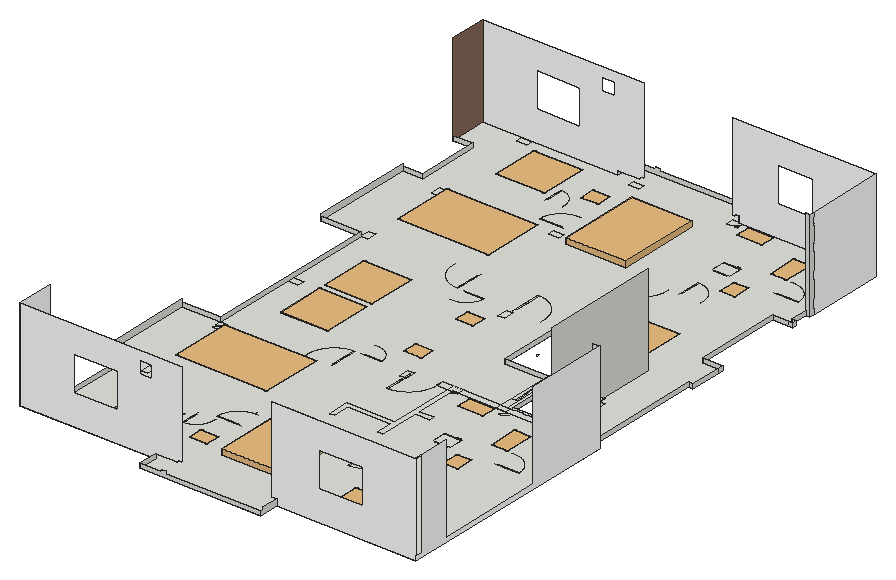
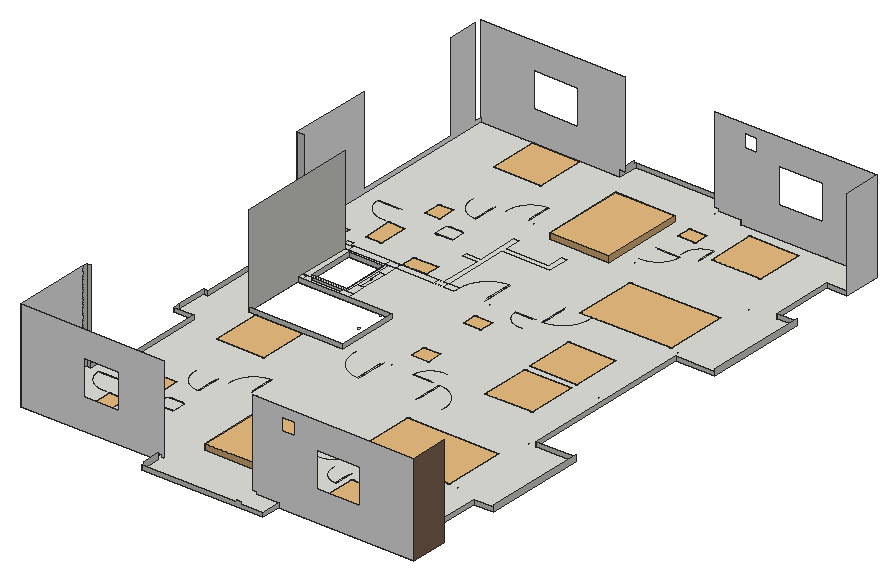
# SketchUp Ruby script. Lengths in inches.
U = 1.inch
M = Sketchup.active_model
def pt(a) = Geom::Point3d.new(a.map { |v| v * U })
def face(e, loops, mat)
  f = e.add_face(loops[0].map { |a| pt(a) })
  loops[1..].each { |l| e.add_face(l.map { |a| pt(a) }).erase! }
  f.material = f.back_material = mat if mat
  f
end
# faces: each face lists its corners as indices into pts; further lists are holes
def faces(e, pts, list, mat = nil) = list.each { |f| face(e, (f[0].is_a?(Array) ? f : [f]).map { |l| l.map { |i| pts[i] } }, mat) }
# xy, xz, yz: faces in a plane at the given z, y or x. An outline is a flat list of corners, or four numbers for a rectangle; further outlines are holes
def ring(l) = l.size == 4 ? [[l[0], l[1]], [l[2], l[1]], [l[2], l[3]], [l[0], l[3]]] : l.each_slice(2).to_a
def flat(e, list, mat, &to3) = list.each { |f| face(e, (f[0].is_a?(Array) ? f : [f]).map { |l| ring(l).map { |u, v| to3.(u, v) } }, mat) }
def xy(e, z, list, mat = nil) = flat(e, list, mat) { |x, y| [x, y, z] }
def xz(e, y, list, mat = nil) = flat(e, list, mat) { |x, z| [x, y, z] }
def yz(e, x, list, mat = nil) = flat(e, list, mat) { |y, z| [x, y, z] }
def lines(e, pts, list) = list.each { |a, b| e.add_line(pt(pts[a]), pt(pts[b])) }
# prism: a flat outline (further loops are holes) pulled along v
def prism(e, loops, v, mat = nil)
  f = face(e, loops, mat); d = Geom::Vector3d.new(v.map { |x| x * U })
  f.pushpull(f.normal.samedirection?(d) ? d.length : -d.length)
end
def box(e, o, s, mat = nil) = prism(e, [[o, [o[0] + s[0], o[1], o[2]], [o[0] + s[0], o[1] + s[1], o[2]], [o[0], o[1] + s[1], o[2]]]], [0, 0, s[2]], mat)
def at(x, y, z, deg = 0) = Geom::Transformation.translation(pt([x, y, z])) * Geom::Transformation.rotation(ORIGIN, Z_AXIS, deg.degrees)
def axes(o, x, y, z) = Geom::Transformation.new([*x, 0, *y, 0, *z, 0, *pt(o).to_a, 1])
def part(name) = M.definitions.add(name)
# library, detail: a bought-in or finely detailed component or shape, given as its bounding box
def library(name, o, s) = part(name).tap { |d| box(d.entities, o, s) }
def detail(e, o, s) = box(e.add_group.entities, o, s)
def put(e, d, t, mat = nil) = e.add_instance(d, t).tap { |i| i.material = mat if mat }
def group(e, t, mat = nil) = e.add_group.tap { |g| g.transformation = t; g.material = mat if mat }.entities
root = M.entities
M.materials.add("Manhattan Creative Coating ML 1016B 24.75cm").color = [255, 255, 255]
M.materials.add("Wood Planks C01 100cm\#1").color = [136, 107, 89]
c1 = library("A$C403C54AD\#3",[0,0,-0.17],[8.08,5.86,0.57])
c2 = library("TARJA2\#3",[-2.49,-4.93,0],[8.71,4.91,0.01])
c3 = part("A$C42203764\#3")
put(c3.entities,c2,axes([263.32,520.21,0],[105.57605,0,0],[0,105.57605,0],[0,0,105.57605]))
c4 = library("A$C038F079D\#3",[0,0,0],[750,440,0.01])
c5 = library("A$C00C51FE0\#3",[0,0,0],[20,24.125,0.01])
c6 = library("A$C20C229D7\#3",[0,576,0],[24,24,0.01])
c7 = part("A$C659B0DF6\#3")
p = [[21.05,606.07,0],[21.05,607.55,0],[17.35,607.55,0],[17.35,606.07,0],[24,604.22,0],[0,604.22,0],
  [24,606.07,0],[0,606.07,0],[20.625,583.91,0],[20.625,585.72,0],[3.375,583.91,0],[3.375,585.72,0],
  [0,585.72,0],[24,585.72,0]]
lines(c7.entities,p,[[0,1],[2,3],[1,2],[4,5],[6,7],[8,9],[10,11],[10,8],[12,7],[13,6],[13,12]])
c8 = library("A$C4DC51D13\#3",[-0.71,0,0],[4438.2,2996.1875,0.01])
c9 = library("A$C52B64FF5\#3",[0,0,0],[6.95,7.1875,0.01])
c10 = part("*U13\#3")
p = [[0,0,0],[0,24,0],[-1.75,24,0],[-1.75,0,0],[-1.57,23.95,0],[-3.13,23.79,0],
  [-4.68,23.54,0],[-6.21,23.18,0],[-7.71,22.73,0],[-9.18,22.17,0],[-10.61,21.52,0],[-12,20.78,0],
  [-13.33,19.96,0],[-14.61,19.04,0],[-15.82,18.04,0],[-16.97,16.97,0],[-18.04,15.82,0],[-19.04,14.61,0],
  [-19.96,13.33,0],[-20.78,12,0],[-21.52,10.61,0],[-22.17,9.18,0],[-22.73,7.71,0],[-23.18,6.21,0],
  [-23.54,4.68,0],[-23.79,3.13,0],[-23.95,1.57,0],[-24,0,0],[0,-4,0],[-24,-4,0]]
lines(c10.entities,p,[[0,1],[1,2],[2,3],[3,0],[1,4],[4,5],[5,6],[6,7],[7,8],[8,9],[9,10],[10,11],
  [11,12],[12,13],[13,14],[14,15],[15,16],[16,17],[17,18],[18,19],[19,20],[20,21],[21,22],[22,23],
  [23,24],[24,25],[25,26],[26,27],[0,28],[27,29]])
c11 = part("*U14\#3")
p = [[0,0,0],[0,24,0],[1.75,24,0],[1.75,0,0],[24,0,0],[23.95,1.51,0],
  [23.8125,3.01,0],[23.57,4.5,0],[23.25,5.97,0],[22.83,7.42,0],[22.31,8.83,0],[21.72,10.22,0],
  [21.03,11.5625,0],[20.26,12.86,0],[19.42,14.11,0],[18.49,15.3,0],[17.5,16.43,0],[16.43,17.5,0],
  [15.3,18.49,0],[14.11,19.42,0],[12.86,20.26,0],[11.5625,21.03,0],[10.22,21.72,0],[8.83,22.31,0],
  [7.42,22.83,0],[5.97,23.25,0],[4.5,23.57,0],[3.01,23.8125,0],[1.51,23.95,0],[0,-4,0],
  [24,-4,0]]
lines(c11.entities,p,[[0,1],[1,2],[2,3],[3,0],[4,5],[5,6],[6,7],[7,8],[8,9],[9,10],[10,11],[11,12],
  [12,13],[13,14],[14,15],[15,16],[16,17],[17,18],[18,19],[19,20],[20,21],[21,22],[22,23],[23,24],
  [24,25],[25,26],[26,27],[27,28],[28,1],[0,29],[4,30]])
c12 = part("*U15\#3")
p = [[0,0,0],[0,30,0],[-1.75,30,0],[-1.75,0,0],[-1.96,29.9375,0],[-3.92,29.74,0],
  [-5.85,29.42,0],[-7.76,28.98,0],[-9.64,28.41,0],[-11.48,27.72,0],[-13.27,26.91,0],[-15,25.98,0],
  [-16.67,24.94,0],[-18.26,23.8,0],[-19.78,22.56,0],[-21.21,21.21,0],[-22.56,19.78,0],[-23.8,18.26,0],
  [-24.94,16.67,0],[-25.98,15,0],[-26.91,13.27,0],[-27.72,11.48,0],[-28.41,9.64,0],[-28.98,7.76,0],
  [-29.42,5.85,0],[-29.74,3.92,0],[-29.9375,1.96,0],[-30,0,0],[0,-4,0],[-30,-4,0]]
lines(c12.entities,p,[[0,1],[1,2],[2,3],[3,0],[1,4],[4,5],[5,6],[6,7],[7,8],[8,9],[9,10],[10,11],
  [11,12],[12,13],[13,14],[14,15],[15,16],[16,17],[17,18],[18,19],[19,20],[20,21],[21,22],[22,23],
  [23,24],[24,25],[25,26],[26,27],[0,28],[27,29]])
c13 = part("*U12\#3")
p = [[0,0,0],[0,-30,0],[-1.75,-30,0],[-1.75,0,0],[-30,0,0],[-29.94,-1.88,0],
  [-29.76,-3.76,0],[-29.47,-5.62,0],[-29.06,-7.46,0],[-28.53,-9.27,0],[-27.89,-11.04,0],[-27.14,-12.77,0],
  [-26.29,-14.45,0],[-25.33,-16.07,0],[-24.27,-17.63,0],[-23.12,-19.12,0],[-21.87,-20.54,0],[-20.54,-21.87,0],
  [-19.12,-23.12,0],[-17.63,-24.27,0],[-16.07,-25.33,0],[-14.45,-26.29,0],[-12.77,-27.14,0],[-11.04,-27.89,0],
  [-9.27,-28.53,0],[-7.46,-29.06,0],[-5.62,-29.47,0],[-3.76,-29.76,0],[-1.88,-29.94,0],[0,4,0],
  [-30,4,0]]
lines(c13.entities,p,[[0,1],[1,2],[2,3],[3,0],[4,5],[5,6],[6,7],[7,8],[8,9],[9,10],[10,11],[11,12],
  [12,13],[13,14],[14,15],[15,16],[16,17],[17,18],[18,19],[19,20],[20,21],[21,22],[22,23],[23,24],
  [24,25],[25,26],[26,27],[27,28],[28,1],[0,29],[4,30]])
c14 = part("*U9\#3")
p = [[0,0,0],[0,36,0],[-1.75,36,0],[-1.75,0,0],[-2.35,35.92,0],[-4.7,35.69,0],
  [-7.02,35.31,0],[-9.32,34.77,0],[-11.57,34.09,0],[-13.78,33.26,0],[-15.92,32.29,0],[-18,31.18,0],
  [-20,29.93,0],[-21.92,28.5625,0],[-23.74,27.07,0],[-25.46,25.46,0],[-27.07,23.74,0],[-28.5625,21.92,0],
  [-29.93,20,0],[-31.18,18,0],[-32.29,15.92,0],[-33.26,13.78,0],[-34.09,11.57,0],[-34.77,9.32,0],
  [-35.31,7.02,0],[-35.69,4.7,0],[-35.92,2.35,0],[-36,0,0],[0,-4,0],[-36,-4,0]]
lines(c14.entities,p,[[0,1],[1,2],[2,3],[3,0],[1,4],[4,5],[5,6],[6,7],[7,8],[8,9],[9,10],[10,11],
  [11,12],[12,13],[13,14],[14,15],[15,16],[16,17],[17,18],[18,19],[19,20],[20,21],[21,22],[22,23],
  [23,24],[24,25],[25,26],[26,27],[0,28],[27,29]])
c15 = part("*U8\#3")
p = [[0,0,0],[0,-36,0],[-1.75,-36,0],[-1.75,0,0],[-36,0,0],[-35.93,-2.26,0],
  [-35.72,-4.51,0],[-35.36,-6.75,0],[-34.87,-8.95,0],[-34.24,-11.125,0],[-33.47,-13.25,0],[-32.57,-15.33,0],
  [-31.55,-17.34,0],[-30.4,-19.29,0],[-29.125,-21.16,0],[-27.74,-22.95,0],[-26.24,-24.64,0],[-24.64,-26.24,0],
  [-22.95,-27.74,0],[-21.16,-29.125,0],[-19.29,-30.4,0],[-17.34,-31.55,0],[-15.33,-32.57,0],[-13.25,-33.47,0],
  [-11.125,-34.24,0],[-8.95,-34.87,0],[-6.75,-35.36,0],[-4.51,-35.72,0],[-2.26,-35.93,0],[0,4,0],
  [-36,4,0]]
lines(c15.entities,p,[[0,1],[1,2],[2,3],[3,0],[4,5],[5,6],[6,7],[7,8],[8,9],[9,10],[10,11],[11,12],
  [12,13],[13,14],[14,15],[15,16],[16,17],[17,18],[18,19],[19,20],[20,21],[21,22],[22,23],[23,24],
  [24,25],[25,26],[26,27],[27,28],[28,1],[0,29],[4,30]])
c16 = part("*U7\#3")
p = [[0,0,0],[0,24,0],[1.75,24,0],[1.75,0,0],[24,0,0],[23.95,1.51,0],
  [23.8125,3.01,0],[23.57,4.5,0],[23.25,5.97,0],[22.83,7.42,0],[22.31,8.83,0],[21.72,10.22,0],
  [21.03,11.5625,0],[20.26,12.86,0],[19.42,14.11,0],[18.49,15.3,0],[17.5,16.43,0],[16.43,17.5,0],
  [15.3,18.49,0],[14.11,19.42,0],[12.86,20.26,0],[11.5625,21.03,0],[10.22,21.72,0],[8.83,22.31,0],
  [7.42,22.83,0],[5.97,23.25,0],[4.5,23.57,0],[3.01,23.8125,0],[1.51,23.95,0],[0,-4,0],
  [24,-4,0]]
lines(c16.entities,p,[[0,1],[1,2],[2,3],[3,0],[4,5],[5,6],[6,7],[7,8],[8,9],[9,10],[10,11],[11,12],
  [12,13],[13,14],[14,15],[15,16],[16,17],[17,18],[18,19],[19,20],[20,21],[21,22],[22,23],[23,24],
  [24,25],[25,26],[26,27],[27,28],[28,1],[0,29],[4,30]])
c17 = part("*U6\#3")
p = [[0,0,0],[0,-24,0],[1.75,-24,0],[1.75,0,0],[1.51,-23.95,0],[3.01,-23.8125,0],
  [4.5,-23.57,0],[5.97,-23.25,0],[7.42,-22.83,0],[8.83,-22.31,0],[10.22,-21.72,0],[11.5625,-21.03,0],
  [12.86,-20.26,0],[14.11,-19.42,0],[15.3,-18.49,0],[16.43,-17.5,0],[17.5,-16.43,0],[18.49,-15.3,0],
  [19.42,-14.11,0],[20.26,-12.86,0],[21.03,-11.5625,0],[21.72,-10.22,0],[22.31,-8.83,0],[22.83,-7.42,0],
  [23.25,-5.97,0],[23.57,-4.5,0],[23.8125,-3.01,0],[23.95,-1.51,0],[24,0,0],[0,4,0],
  [24,4,0]]
lines(c17.entities,p,[[0,1],[1,2],[2,3],[3,0],[1,4],[4,5],[5,6],[6,7],[7,8],[8,9],[9,10],[10,11],
  [11,12],[12,13],[13,14],[14,15],[15,16],[16,17],[17,18],[18,19],[19,20],[20,21],[21,22],[22,23],
  [23,24],[24,25],[25,26],[26,27],[27,28],[0,29],[28,30]])
c18 = part("*U5\#3")
p = [[0,0,0],[0,-28,0],[1.75,-28,0],[1.75,0,0],[1.76,-27.94,0],[3.51,-27.78,0],
  [5.25,-27.5,0],[6.96,-27.12,0],[8.65,-26.63,0],[10.31,-26.03,0],[11.92,-25.34,0],[13.49,-24.54,0],
  [15,-23.64,0],[16.46,-22.65,0],[17.85,-21.57,0],[19.17,-20.41,0],[20.41,-19.17,0],[21.57,-17.85,0],
  [22.65,-16.46,0],[23.64,-15,0],[24.54,-13.49,0],[25.34,-11.92,0],[26.03,-10.31,0],[26.63,-8.65,0],
  [27.12,-6.96,0],[27.5,-5.25,0],[27.78,-3.51,0],[27.94,-1.76,0],[28,0,0],[0,4,0],
  [28,4,0]]
lines(c18.entities,p,[[0,1],[1,2],[2,3],[3,0],[1,4],[4,5],[5,6],[6,7],[7,8],[8,9],[9,10],[10,11],
  [11,12],[12,13],[13,14],[14,15],[15,16],[16,17],[17,18],[18,19],[19,20],[20,21],[21,22],[22,23],
  [23,24],[24,25],[25,26],[26,27],[27,28],[0,29],[28,30]])
c19 = part("*U4\#3")
p = [[0,0,0],[0,28,0],[1.75,28,0],[1.75,0,0],[28,0,0],[27.94,1.76,0],
  [27.78,3.51,0],[27.5,5.25,0],[27.12,6.96,0],[26.63,8.65,0],[26.03,10.31,0],[25.34,11.92,0],
  [24.54,13.49,0],[23.64,15,0],[22.65,16.46,0],[21.57,17.85,0],[20.41,19.17,0],[19.17,20.41,0],
  [17.85,21.57,0],[16.46,22.65,0],[15,23.64,0],[13.49,24.54,0],[11.92,25.34,0],[10.31,26.03,0],
  [8.65,26.63,0],[6.96,27.12,0],[5.25,27.5,0],[3.51,27.78,0],[1.76,27.94,0],[0,-4,0],
  [28,-4,0]]
lines(c19.entities,p,[[0,1],[1,2],[2,3],[3,0],[4,5],[5,6],[6,7],[7,8],[8,9],[9,10],[10,11],[11,12],
  [12,13],[13,14],[14,15],[15,16],[16,17],[17,18],[18,19],[19,20],[20,21],[21,22],[22,23],[23,24],
  [24,25],[25,26],[26,27],[27,28],[28,1],[0,29],[4,30]])
c20 = part("*U3\#3")
p = [[0,0,0],[0,30,0],[1.75,30,0],[1.75,0,0],[30,0,0],[29.94,1.88,0],
  [29.76,3.76,0],[29.47,5.62,0],[29.06,7.46,0],[28.53,9.27,0],[27.89,11.04,0],[27.14,12.77,0],
  [26.29,14.45,0],[25.33,16.07,0],[24.27,17.63,0],[23.12,19.12,0],[21.87,20.54,0],[20.54,21.87,0],
  [19.12,23.12,0],[17.63,24.27,0],[16.07,25.33,0],[14.45,26.29,0],[12.77,27.14,0],[11.04,27.89,0],
  [9.27,28.53,0],[7.46,29.06,0],[5.62,29.47,0],[3.76,29.76,0],[1.88,29.94,0],[0,-4,0],
  [30,-4,0]]
lines(c20.entities,p,[[0,1],[1,2],[2,3],[3,0],[4,5],[5,6],[6,7],[7,8],[8,9],[9,10],[10,11],[11,12],
  [12,13],[13,14],[14,15],[15,16],[16,17],[17,18],[18,19],[19,20],[20,21],[21,22],[22,23],[23,24],
  [24,25],[25,26],[26,27],[27,28],[28,1],[0,29],[4,30]])
c21 = part("*U2\#3")
p = [[0,0,0],[0,-32,0],[1.75,-32,0],[1.75,0,0],[2.01,-31.9375,0],[4.01,-31.75,0],
  [6,-31.43,0],[7.96,-30.99,0],[9.89,-30.43,0],[11.78,-29.75,0],[13.625,-28.95,0],[15.42,-28.04,0],
  [17.15,-27.02,0],[18.81,-25.89,0],[20.4,-24.66,0],[21.91,-23.33,0],[23.33,-21.91,0],[24.66,-20.4,0],
  [25.89,-18.81,0],[27.02,-17.15,0],[28.04,-15.42,0],[28.95,-13.625,0],[29.75,-11.78,0],[30.43,-9.89,0],
  [30.99,-7.96,0],[31.43,-6,0],[31.75,-4.01,0],[31.9375,-2.01,0],[32,0,0],[0,4,0],
  [32,4,0]]
lines(c21.entities,p,[[0,1],[1,2],[2,3],[3,0],[1,4],[4,5],[5,6],[6,7],[7,8],[8,9],[9,10],[10,11],
  [11,12],[12,13],[13,14],[14,15],[15,16],[16,17],[17,18],[18,19],[19,20],[20,21],[21,22],[22,23],
  [23,24],[24,25],[25,26],[26,27],[27,28],[0,29],[28,30]])
c22 = part("Commercial Building Flr Plans.dwg\#3")
xy(c22.entities,0,[[722.01,373.53,728.01,373.53,728.01,396.03,788.01,396.03,788.01,373.53,794.01,373.53,794.01,430.53,814.01,430.53,814.01,436.53,794.01,436.53,794.01,493.53,923.01,493.53,923.01,487.53,932.01,487.53,932.01,493.53,918.01,493.53,918.01,502.53,868.01,502.53,868.01,493.53,854.01,493.53,854.01,502.53,773.01,502.53,773.01,493.53,788.01,493.53,788.01,502.53,802.01,502.53,802.01,493.53,788.01,493.53,788.01,402.03,722.01,402.03],[854.01,493.53,868.01,502.53],[918.01,493.53,932.01,502.53],[854.01,502.53,863.01,520.53],[[863.01,502.53,923.01,574.53],[867.01,506.53,915.01,570.53]],
  [923.01,502.53,932.01,502.53,932.01,583.53,932.01,574.53,923.01,574.53],[854.01,520.53,859.01,520.53,859.01,538.53,858.01,538.53,858.01,556.53,854.01,556.53],[859.01,520.53,860.01,538.53],[860.01,520.53,863.01,520.53,863.01,556.53,859.01,556.53,859.01,538.53,860.01,538.53],[858.01,538.53,859.01,556.53],
  [854.01,556.53,863.01,574.53],[854.01,574.53,868.01,583.53],[918.01,574.53,932.01,583.53]])
xz(c22.entities,506.53,[[867.01,-6,915.01,0]])
xz(c22.entities,570.53,[[867.01,-6,915.01,0]])
yz(c22.entities,867.01,[[506.53,-6,570.53,0]])
yz(c22.entities,915.01,[[506.53,-6,570.53,0]])
# 5414 loose lines left out
put(c22.entities,c1,axes([684.95,938.32,0.02],[0,-14.03023,0],[14.03023,0,0],[0,0,14.03023]))
put(c22.entities,c1,axes([684.95,346.29,0.02],[0,-14.03023,0],[14.03023,0,0],[0,0,14.03023]))
put(c22.entities,c3,axes([900.04,908.53,0],[0,0.04349,0],[0.04349,0,0],[0,0,0.04349]))
put(c22.entities,c3,axes([900.04,428.53,0],[0,0.04349,0],[0.04349,0,0],[0,0,0.04349]))
put(c22.entities,c4,axes([819.23,471.91,0],[0.04545,0,0],[0,0.04545,0],[0,0,0.04545]))
put(c22.entities,c4,axes([819.23,951.91,0],[0.04545,0,0],[0,0.04545,0],[0,0,0.04545]))
put(c22.entities,c5,axes([722.01,550.53,0],[0,-1,0],[-1,0,0],[0,0,1]))
put(c22.entities,c5,at(660.51,238.53,0,90))
put(c22.entities,c5,at(722.01,619.53,0,90))
put(c22.entities,c5,at(660.51,911.53,0,90))
put(c22.entities,c5,at(901.51,868.5,0,180))
put(c22.entities,c5,at(904.51,388.5,0,180))
put(c22.entities,c6,at(942.55,371.21,0))
put(c22.entities,c6,at(945.55,-108.79,0))
put(c22.entities,c7,at(845.01,-189.39,0))
put(c22.entities,c7,at(845.01,290.61,0))
put(c22.entities,c8,axes([512.64,369.84,0],[0.02827,0,0],[0,0.02827,0],[0,0,0.02827]))
put(c22.entities,c8,axes([512.64,750.84,0],[0.02827,0,0],[0,0.02827,0],[0,0,0.02827]))
put(c22.entities,c9,axes([533.03,959.68,0],[0,-9.39007,0],[9.39007,0,0],[0,0,9.39007]))
put(c22.entities,c9,axes([841.85,744,0],[9.39007,0,0],[0,-9.39007,0],[0,0,9.39007]))
put(c22.entities,c9,axes([844.85,264,0],[9.39007,0,0],[0,-9.39007,0],[0,0,9.39007]))
put(c22.entities,c9,axes([541.85,657,0],[9.39007,0,0],[0,-9.39007,0],[0,0,9.39007]))
put(c22.entities,c9,axes([541.85,513.06,0],[9.39007,0,0],[0,9.39007,0],[0,0,9.39007]))
put(c22.entities,c9,axes([533.03,275.68,0],[0,-9.39007,0],[9.39007,0,0],[0,0,9.39007]))
put(c22.entities,c10,at(669.51,496.53,0,-90))
put(c22.entities,c11,at(669.51,673.53,0,-90))
put(c22.entities,c12,at(932.01,397.53,0,-90))
put(c22.entities,c12,at(932.01,877.53,0,-90))
put(c22.entities,c13,at(660.51,292.53,0,-90))
put(c22.entities,c13,at(660.51,847.03,0,-90))
put(c22.entities,c14,at(657.51,460.53,0))
put(c22.entities,c15,at(657.51,709.53,0))
put(c22.entities,c16,at(609.51,886.53,0))
put(c22.entities,c17,at(609.51,283.53,0))
put(c22.entities,c18,axes([734.01,493.53,0],[1.39286,0,0],[0,1.39286,0],[0,0,1.39286]))
put(c22.entities,c19,axes([734.01,676.53,0],[1.39286,0,0],[0,1.39286,0],[0,0,1.39286]))
put(c22.entities,c20,at(854.01,334.53,0))
put(c22.entities,c20,at(851.01,814.53,0))
put(c22.entities,c21,at(807.51,328.53,0))
put(c22.entities,c21,at(804.51,808.53,0))
xy(root,119.7,[[2153.41,896.68,2153.67,896.68,2153.92,896.76,2154.15,896.89,2154.33,897.08,2154.45,897.31,2154.52,897.56,2154.51,897.82,2154.44,898.07,2154.31,898.3,2154.12,898.48,2153.89,898.6,2153.64,898.67,2153.38,898.66,2153.125,898.59,2152.9,898.46,2152.72,898.27,2152.59,898.04,2152.53,897.79,2152.53,897.53,2152.61,897.28,2152.74,897.05,2152.93,896.87,2153.16,896.74],[2153.41,933.68,2153.67,933.68,2153.92,933.76,2154.15,933.89,2154.33,934.08,2154.45,934.31,2154.52,934.56,2154.51,934.82,2154.44,935.07,2154.31,935.3,2154.12,935.48,2153.89,935.6,2153.64,935.67,2153.38,935.66,2153.125,935.59,2152.9,935.46,2152.72,935.27,2152.59,935.04,2152.53,934.79,2152.53,934.53,2152.61,934.28,2152.74,934.05,2152.93,933.87,2153.16,933.74]])
xy(root,120,[[[1975.05,473.67,1975.05,500.67,1789.02,500.67,1789.02,551.67,1816.02,551.67,1816.02,637.17,1789.02,637.17,1789.02,778.17,1843.02,778.17,1843.02,1018.17,1789.02,1018.17,1789.02,1159.17,1816.02,1159.17,1816.02,1244.67,1789.02,1244.67,1789.02,1295.67,1975.05,1295.67,1975.05,1322.67,2141.52,1322.67,2141.52,1295.67,2330.52,1295.67,2330.52,1181.67,2324.52,1181.67,2324.52,1157.7,2330.52,1157.7,2330.52,1151.7,2303.52,1151.7,2303.52,1031.67,2330.52,1031.67,2330.52,980.67,2324.52,980.67,2324.52,815.67,2333.52,815.67,2333.52,500.67,2141.52,500.67,2141.52,473.67],[2138.52,896.67,2267.52,980.67],[2211.52,819.67,2259.52,883.67]],[1843.02,500.67,1857.02,509.67],[1997.02,500.67,2011.02,509.67],[2135.52,500.67,2149.52,509.67],[2262.52,500.67,2276.52,509.67],
  [1997.02,638.67,2011.02,647.67],[2135.52,638.67,2149.52,647.67],[1843.02,641.67,1852.02,655.67],[1843.02,763.67,1852.02,777.67],[2066.52,806.67,2075.52,820.67],
  [2132.52,806.67,2146.52,815.67],[2198.52,806.67,2212.52,815.67],[2262.52,806.67,2276.52,815.67],[2262.52,819.67,2276.52,896.67],[1843.02,893.67,1857.02,902.67],
  [2066.52,975.67,2075.52,989.67],[2132.52,980.67,2146.52,1061.67],[1843.02,1018.67,1852.02,1032.67],[2132.52,1118.67,2146.52,1127.67],[1843.02,1140.67,1852.02,1154.67],
  [1997.02,1148.67,2011.02,1157.67],[1843.02,1286.67,1857.02,1295.67],[1997.02,1286.67,2011.02,1295.67],[2132.52,1286.67,2146.52,1295.67],[2262.52,1286.67,2276.52,1295.67]])
xz(root,473.67,[[1975.05,120,2141.52,120,2141.52,126,2011.02,126,2011.02,129,2005.02,129,2005.02,126,1975.05,126]])
xz(root,500.67,[[[1789.02,120,1975.05,120,1975.05,126,2005.02,126,2005.02,129,2011.02,129,2011.02,246,1789.02,246],[1863.02,162,1923.02,210],[1953.02,216,1970.52,234]],[[2141.52,120,2333.52,120,2333.52,246,2135.52,246,2135.52,129,2141.52,129],[2199.52,162,2259.52,210]]],"Manhattan Creative Coating ML 1016B 24.75cm")
xz(root,551.67,[[1789.02,120,1816.02,126]])
xz(root,637.17,[[1789.02,120,1816.02,126]])
xz(root,778.17,[[1789.02,120,1843.02,126]])
xz(root,815.67,[[2324.52,120,2333.52,246]])
xz(root,896.67,[[2138.52,120,2267.52,126]])
xz(root,980.67,[[2138.52,120,2267.52,126],[2324.52,120,2330.52,126]])
xz(root,1018.17,[[1789.02,120,1843.02,126]])
xz(root,1031.67,[[2303.52,120,2330.52,126]])
xz(root,1151.7,[[2303.52,120,2324.52,126],[2324.52,120,2330.52,126]])
xz(root,1157.7,[[2324.52,120,2330.52,126]])
xz(root,1159.17,[[1789.02,120,1816.02,126]])
xz(root,1181.67,[[2324.52,120,2330.52,246]])
xz(root,1244.67,[[1789.02,120,1816.02,126]])
xz(root,1295.67,[[[1789.02,120,1789.02,246,2011.02,246,2011.02,129,2005.02,129,2005.02,126,1975.05,126,1975.05,120],[1863.02,162,1923.02,210],[1953.02,216,1970.52,234]],[[2141.52,120,2141.52,129,2135.52,129,2135.52,126,2132.52,126,2132.52,246,2330.52,246,2330.52,120],[2195.52,162,2243.52,210]]],"Manhattan Creative Coating ML 1016B 24.75cm")
xz(root,1322.67,[[1975.05,120,1975.05,126,2005.02,126,2005.02,129,2011.02,129,2011.02,126,2141.52,126,2141.52,120]])
yz(root,1789.02,[[637.17,120,778.17,129],[1018.17,120,1159.17,129]])
yz(root,1789.02,[[500.67,120,551.67,246]],"Manhattan Creative Coating ML 1016B 24.75cm")
yz(root,1789.02,[[1244.67,120,1295.67,246]],"Wood Planks C01 100cm\#1")
yz(root,1816.02,[[551.67,120,637.17,126],[1159.17,120,1244.67,126]])
yz(root,1843.02,[[778.17,120,1018.17,126]])
yz(root,1975.05,[[473.67,120,500.67,126],[1295.67,120,1322.67,126]])
yz(root,2138.52,[[896.67,120,980.67,126]])
yz(root,2141.52,[[473.67,120,500.67,120,500.67,129,476.67,129,476.67,126,473.67,126],[1295.67,120,1322.67,120,1322.67,126,1319.67,126,1319.67,129,1295.67,129]])
yz(root,2267.52,[[896.67,120,896.67,126,815.67,126,815.67,246,980.67,246,980.67,120]])
yz(root,2303.52,[[1031.67,120,1151.7,126]])
yz(root,2324.52,[[815.67,120,980.67,126],[1157.7,120,1181.67,126]])
yz(root,2330.52,[[980.67,120,1022.67,126],[1022.67,120,1031.67,126],[1151.7,120,1157.7,126],[1181.67,120,1187.67,246]])
yz(root,2330.52,[[1187.67,120,1295.67,246]],"Manhattan Creative Coating ML 1016B 24.75cm")
yz(root,2333.52,[[500.67,120,815.67,120,815.67,246,701.67,246,701.67,126,551.67,126,551.67,246,509.67,246,509.67,126,500.67,126]],"Manhattan Creative Coating ML 1016B 24.75cm")
put(root,c22,at(1344.52,313.15,126))
